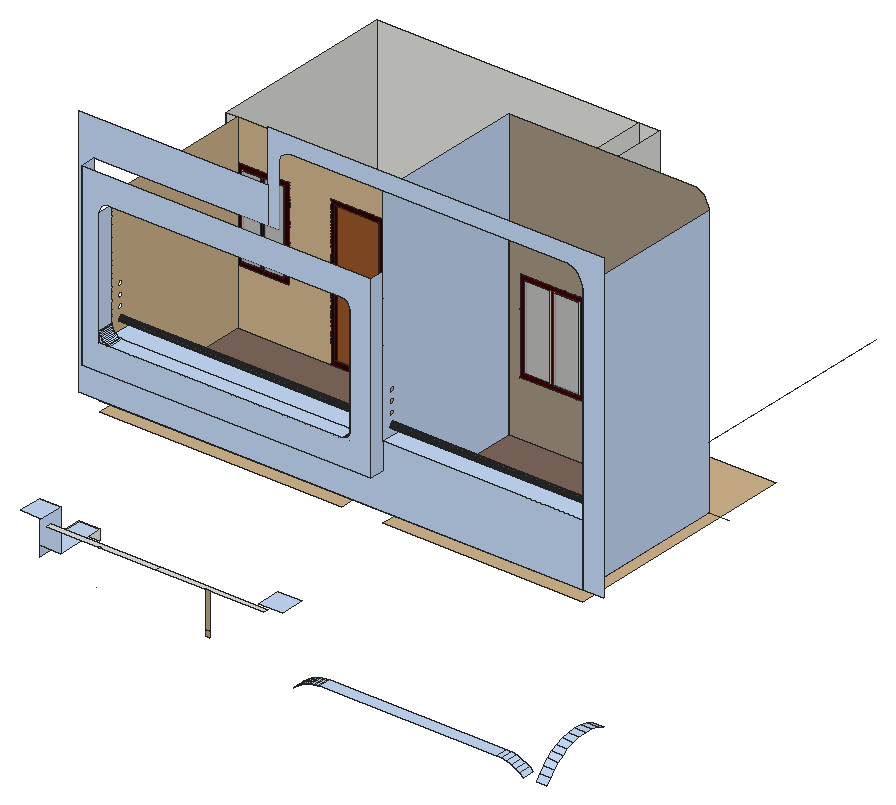
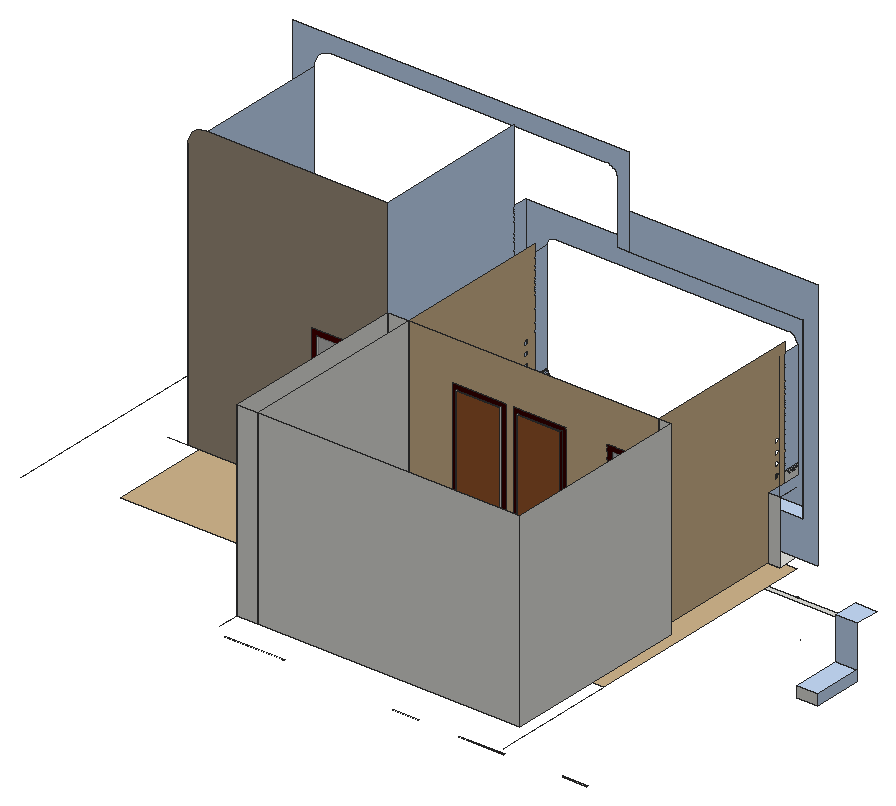
# SketchUp Ruby script. Lengths in inches.
U = 1.inch
M = Sketchup.active_model
def pt(a) = Geom::Point3d.new(a.map { |v| v * U })
def face(e, loops, mat)
  f = e.add_face(loops[0].map { |a| pt(a) })
  loops[1..].each { |l| e.add_face(l.map { |a| pt(a) }).erase! }
  f.material = f.back_material = mat if mat
  f
end
# faces: each face lists its corners as indices into pts; further lists are holes
def faces(e, pts, list, mat = nil) = list.each { |f| face(e, (f[0].is_a?(Array) ? f : [f]).map { |l| l.map { |i| pts[i] } }, mat) }
# xy, xz, yz: faces in a plane at the given z, y or x. An outline is a flat list of corners, or four numbers for a rectangle; further outlines are holes
def ring(l) = l.size == 4 ? [[l[0], l[1]], [l[2], l[1]], [l[2], l[3]], [l[0], l[3]]] : l.each_slice(2).to_a
def flat(e, list, mat, &to3) = list.each { |f| face(e, (f[0].is_a?(Array) ? f : [f]).map { |l| ring(l).map { |u, v| to3.(u, v) } }, mat) }
def xy(e, z, list, mat = nil) = flat(e, list, mat) { |x, y| [x, y, z] }
def xz(e, y, list, mat = nil) = flat(e, list, mat) { |x, z| [x, y, z] }
def yz(e, x, list, mat = nil) = flat(e, list, mat) { |y, z| [x, y, z] }
def lines(e, pts, list) = list.each { |a, b| e.add_line(pt(pts[a]), pt(pts[b])) }
# prism: a flat outline (further loops are holes) pulled along v
def prism(e, loops, v, mat = nil)
  f = face(e, loops, mat); d = Geom::Vector3d.new(v.map { |x| x * U })
  f.pushpull(f.normal.samedirection?(d) ? d.length : -d.length)
end
def box(e, o, s, mat = nil) = prism(e, [[o, [o[0] + s[0], o[1], o[2]], [o[0] + s[0], o[1] + s[1], o[2]], [o[0], o[1] + s[1], o[2]]]], [0, 0, s[2]], mat)
def at(x, y, z, deg = 0) = Geom::Transformation.translation(pt([x, y, z])) * Geom::Transformation.rotation(ORIGIN, Z_AXIS, deg.degrees)
def axes(o, x, y, z) = Geom::Transformation.new([*x, 0, *y, 0, *z, 0, *pt(o).to_a, 1])
def part(name) = M.definitions.add(name)
# library, detail: a bought-in or finely detailed component or shape, given as its bounding box
def library(name, o, s) = part(name).tap { |d| box(d.entities, o, s) }
def detail(e, o, s) = box(e.add_group.entities, o, s)
def put(e, d, t, mat = nil) = e.add_instance(d, t).tap { |i| i.material = mat if mat }
def group(e, t, mat = nil) = e.add_group.tap { |g| g.transformation = t; g.material = mat if mat }.entities
root = M.entities
M.materials.add("[0022_Maroon]").color = [56, 0, 0]
M.materials.add("[0022_Maroon]1").color = [71, 0, 0]
M.materials.add("[0033_NavajoWhite]").color = [209, 182, 141]
M.materials.add("[0033_NavajoWhite]1").color = [188, 164, 128]
M.materials.add("[0099_LightSteelBlue]").color = [198, 220, 249]
M.materials.add("[Cladding Siding Tan]").color = [162, 148, 128]
M.materials.add("[Granite Brown]").color = [126, 104, 91]
M.materials.add("[Metal Steel Textured White]").color = [84, 84, 84]
M.materials.add("[Translucent Resin Crush Gray]").color = [184, 184, 184]
M.materials["[Translucent Resin Crush Gray]"].alpha = 0.8
M.materials.add("[Wood Cherry Original]").color = [152, 86, 42]
xy(root,120,[[342.64,0,545.36,13.78]],"[0099_LightSteelBlue]")
xy(root,132,[[0,27.5625,24,84]],"[0099_LightSteelBlue]")
xy(root,143.8125,[[42.69,359,71.07,360],[236.63,359,265,360]])
xy(root,143.8125,[[137.32,360,188.45,361]],"[0022_Maroon]")
xy(root,152.24,[[388.21,360,456,361]])
xy(root,168,[[24,7.78,148.22,13.78],[148.22,7.78,272.4375,13.78]])
xy(root,180,[[0,0,24,27.5625],[272.4375,0,300,27.5625]],"[0099_LightSteelBlue]")
xy(root,252,[[82.32,129.1,79.97,129.1875,77.73,129.88,75.74,131.13,74.14,132.86,73.05,134.9375,72.53,137.23,72.62,139.58,73.31,141.82,74.57,143.81,76.29,145.4,78.37,146.5,80.66,147.02,83.01,146.93,85.25,146.23,87.24,144.98,88.84,143.26,89.93,141.18,90.45,138.89,90.36,136.54,89.67,134.3,88.41,132.31,86.69,130.71,84.61,129.62],[166.32,129.1,163.97,129.1875,161.73,129.88,159.74,131.13,158.14,132.86,157.05,134.9375,156.53,137.23,156.62,139.58,157.31,141.82,158.57,143.81,160.29,145.4,162.37,146.5,164.66,147.02,167.01,146.93,169.25,146.23,171.24,144.98,172.84,143.26,173.93,141.18,174.45,138.89,174.36,136.54,173.67,134.3,172.41,132.31,170.69,130.71,168.61,129.62],[250.32,129.1,247.97,129.1875,245.73,129.88,243.74,131.13,242.14,132.86,241.05,134.9375,240.53,137.23,240.62,139.58,241.31,141.82,242.57,143.81,244.29,145.4,246.37,146.5,248.66,147.02,251.01,146.93,253.25,146.23,255.24,144.98,256.84,143.26,257.93,141.18,258.45,138.89,258.36,136.54,257.67,134.3,256.41,132.31,254.69,130.71,252.61,129.62],[432.35,130.11,430.02,130.42,427.85,131.32,425.99,132.76,424.56,134.62,423.66,136.79,423.36,139.125,423.67,141.45,424.57,143.62,426,145.49,427.87,146.91,430.04,147.81,432.37,148.11,434.7,147.8,436.87,146.9,438.73,145.47,440.16,143.6,441.05,141.43,441.36,139.1,441.05,136.77,440.15,134.6,438.71,132.74,436.85,131.3125,434.68,130.42],[300,180,348,360]])
xy(root,252,[[[24,84,24,360,300,360,300,180,348,180,348,360,576,360,576,84,348,84,348,104.375,300,104.375,300,84],[166.32,129.1,168.61,129.62,170.69,130.71,172.41,132.31,173.67,134.3,174.36,136.54,174.45,138.89,173.93,141.18,172.84,143.26,171.24,144.98,169.25,146.23,167.01,146.93,164.66,147.02,162.37,146.5,160.29,145.4,158.57,143.81,157.31,141.82,156.62,139.58,156.53,137.23,157.05,134.9375,158.14,132.86,159.74,131.13,161.73,129.88,163.97,129.1875],[82.32,129.1,84.61,129.62,86.69,130.71,88.41,132.31,89.67,134.3,90.36,136.54,90.45,138.89,89.93,141.18,88.84,143.26,87.24,144.98,85.25,146.23,83.01,146.93,80.66,147.02,78.37,146.5,76.29,145.4,74.57,143.81,73.31,141.82,72.62,139.58,72.53,137.23,73.05,134.9375,74.14,132.86,75.74,131.13,77.73,129.88,79.97,129.1875],[250.32,129.1,252.61,129.62,254.69,130.71,256.41,132.31,257.67,134.3,258.36,136.54,258.45,138.89,257.93,141.18,256.84,143.26,255.24,144.98,253.25,146.23,251.01,146.93,248.66,147.02,246.37,146.5,244.29,145.4,242.57,143.81,241.31,141.82,240.62,139.58,240.53,137.23,241.05,134.9375,242.14,132.86,243.74,131.13,245.73,129.88,247.97,129.1875],[432.35,130.11,434.68,130.42,436.85,131.3125,438.71,132.74,440.15,134.6,441.05,136.77,441.36,139.1,441.05,141.43,440.16,143.6,438.73,145.47,436.87,146.9,434.7,147.8,432.37,148.11,430.04,147.81,427.87,146.91,426,145.49,424.57,143.62,423.67,141.45,423.36,139.125,423.66,136.79,424.56,134.62,425.99,132.76,427.85,131.32,430.02,130.42]]],"[0033_NavajoWhite]")
xy(root,264,[[24,84,576,108],[324,108,348,264],[24,264,324,480],[324,264,348,480]])
xy(root,264,[[37.43,108,324,264],[348,108,576,264]],"[Granite Brown]")
xy(root,269,[[148.81,264,198.81,266],[218.18,264,268.18,266]])
xy(root,306,[[17.11,66,348,84]],"[0099_LightSteelBlue]")
xy(root,332.63,[[366.6875,263,395.75,264],[399.75,263,428.8125,264]])
xy(root,334.32,[[43.43,263,65.05,264],[69.05,263,90.68,264]])
xy(root,336,[[37.43,66,49.21,84]])
xy(root,336,[[49.21,66,314.66,84],[37.43,84,324,108],[348,84,576,108]],"[0099_LightSteelBlue]")
xz(root,7.78,[[82.51,168,86.11,168,82.51,168.02]])
xz(root,7.78,[[210.33,120.05,210.33,126.08,209.08,126.22,205.44,126.24,205.44,120.25,208.74,120.23],[210.33,126.08,210.33,168,205.44,168,205.44,126.24,209.08,126.22]],"[0033_NavajoWhite]1")
xz(root,27.5625,[[0,132,24,180]],"[0099_LightSteelBlue]")
xz(root,66,[[[17.11,306,348,510],[37.43,336,37.43,469.26,37.52,470.66,37.79,472.04,38.24,473.37,38.86,474.63,39.64,475.8,40.57,476.85,41.625,477.78,42.79,478.5625,44.05,479.18,45.38,479.63,46.76,479.91,48.16,480,314.66,480,315.88,479.92,317.08,479.68,318.24,479.29,319.33,478.75,320.35,478.07,321.27,477.27,322.07,476.35,322.75,475.33,323.29,474.24,323.68,473.08,323.92,471.88,324,470.66,324,345.34,323.92,344.12,323.68,342.92,323.29,341.76,322.75,340.67,322.07,339.65,321.27,338.73,320.35,337.93,319.33,337.25,318.24,336.71,317.08,336.32,315.88,336.08,314.66,336]],[37.43,336,49.21,336,47.67,336.1,46.16,336.4,44.7,336.9,43.32,337.58,42.04,338.4375,40.88,339.45,39.86,340.61,39,341.89,38.32,343.28,37.83,344.74,37.53,346.25,37.43,347.79]],"[0099_LightSteelBlue]")
xz(root,84,[[0,120,24,132]])
xz(root,84,[[0,264,576,264,576,336,348,336,348,306,17.11,306,17.11,510,216,510,216,552,0,552],[576,264,600,264,600,612,216,612,216,510,228,510,228,577.99,228.13,579.93,228.51,581.84,229.13,583.68,229.99,585.42,231.07,587.04,232.35,588.5,233.8125,589.78,235.43,590.86,237.17,591.72,239.01,592.35,240.92,592.72,242.86,592.85,556.05,592.85,558.65,592.68,561.21,592.17,563.68,591.33,566.02,590.18,568.19,588.73,570.16,587.01,571.875,585.05,573.33,582.875,574.48,580.53,575.32,578.0625,575.83,575.5,576,572.9]],"[0099_LightSteelBlue]")
xz(root,108,[[24,264,37.43,336],[324,264,348,336],[348,264,576,336]])
xz(root,108,[[37.43,264,324,336]],"[0099_LightSteelBlue]")
xz(root,263,[[366.6875,332.63,395.75,427.88],[399.75,332.63,428.8125,427.88],[43.43,334.32,65.05,427.88],[69.05,334.32,90.68,427.88]],"[Translucent Resin Crush Gray]")
xz(root,264,[[24,264,37.43,480],[324,264,348,480]])
xz(root,264,[[[143.81,264,203.81,433.88],[148.81,269,198.81,428.88]],[[213.18,264,273.18,433.88],[218.18,269,268.18,428.88]],[[37.43,328.32,96.68,433.88],[43.43,334.32,90.68,427.88]],[65.05,334.32,69.05,427.88]],"[0022_Maroon]")
xz(root,264,[[[360.6875,326.63,434.8125,433.88],[366.6875,332.63,428.8125,427.88]],[395.75,332.63,399.75,427.88]],"[0022_Maroon]1")
xz(root,264,[[37.43,264,143.81,264,143.81,433.88,203.81,433.88,203.81,264,213.18,264,213.18,433.88,273.18,433.88,273.18,264,324,264,324,480,37.43,480,37.43,433.88,96.68,433.88,96.68,328.32,37.43,328.32]],"[0033_NavajoWhite]")
xz(root,264,[[[348,264,576,264,576,572.9,575.83,575.5,575.32,578.0625,574.48,580.53,573.33,582.875,571.875,585.05,570.16,587.01,568.19,588.73,566.02,590.18,563.68,591.33,561.21,592.17,558.65,592.68,556.05,592.85,348,592.85],[360.6875,326.63,434.8125,433.88]]],"[Cladding Siding Tan]")
xz(root,266,[[148.81,269,198.81,428.88],[218.18,269,268.18,428.88]],"[Wood Cherry Original]")
xz(root,480,[[24,264,324,480],[324,264,348,480]])
yz(root,0,[[27.5625,120,84,132]],"[0099_LightSteelBlue]")
yz(root,17.11,[[66,306,84,510]],"[0099_LightSteelBlue]")
yz(root,24,[[264,264,480,480]])
yz(root,37.43,[[66,336,84,347.79]])
yz(root,37.43,[[[108,264,264,264,264,480,84,480,84,336,108,336],[96,381,95.22,381.1,94.5,381.4,93.88,381.88,93.4,382.5,93.1,383.22,93,384,93.1,384.78,93.4,385.5,93.88,386.12,94.5,386.6,95.22,386.9,96,387,96.78,386.9,97.5,386.6,98.12,386.12,98.6,385.5,98.9,384.78,99,384,98.9,383.22,98.6,382.5,98.12,381.88,97.5,381.4,96.78,381.1],[96,369,95.22,369.1,94.5,369.4,93.88,369.88,93.4,370.5,93.1,371.22,93,372,93.1,372.78,93.4,373.5,93.88,374.12,94.5,374.6,95.22,374.9,96,375,96.78,374.9,97.5,374.6,98.12,374.12,98.6,373.5,98.9,372.78,99,372,98.9,371.22,98.6,370.5,98.12,369.88,97.5,369.4,96.78,369.1],[96,357,95.22,357.1,94.5,357.4,93.88,357.88,93.4,358.5,93.1,359.22,93,360,93.1,360.78,93.4,361.5,93.88,362.12,94.5,362.6,95.22,362.9,96,363,96.78,362.9,97.5,362.6,98.12,362.12,98.6,361.5,98.9,360.78,99,360,98.9,359.22,98.6,358.5,98.12,357.88,97.5,357.4,96.78,357.1],[96,345,95.22,345.1,94.5,345.4,93.88,345.88,93.4,346.5,93.1,347.22,93,348,93.1,348.78,93.4,349.5,93.88,350.12,94.5,350.6,95.22,350.9,96,351,96.78,350.9,97.5,350.6,98.12,350.12,98.6,349.5,98.9,348.78,99,348,98.9,347.22,98.6,346.5,98.12,345.88,97.5,345.4,96.78,345.1]]],"[0033_NavajoWhite]")
yz(root,37.43,[[66,347.79,84,469.26]],"[0099_LightSteelBlue]")
yz(root,43.43,[[263,334.32,264,427.88]])
yz(root,65.05,[[263,334.32,264,427.88]],"[0022_Maroon]")
yz(root,69.05,[[263,334.32,264,427.88]])
yz(root,90.68,[[263,334.32,264,427.88]],"[0022_Maroon]")
yz(root,148.81,[[264,269,266,428.88]],"[0022_Maroon]")
yz(root,198.81,[[264,269,266,428.88]])
yz(root,218.18,[[264,269,266,428.88]])
yz(root,268.18,[[264,269,266,428.88]])
yz(root,324,[[264,264,480,480],[96,345,96.78,345.1,97.5,345.4,98.12,345.88,98.6,346.5,98.9,347.22,99,348,98.9,348.78,98.6,349.5,98.12,350.12,97.5,350.6,96.78,350.9,96,351,95.22,350.9,94.5,350.6,93.88,350.12,93.4,349.5,93.1,348.78,93,348,93.1,347.22,93.4,346.5,93.88,345.88,94.5,345.4,95.22,345.1]])
yz(root,324,[[[108,264,108,336,84,336,84,480,264,480,264,264],[96,369,96.78,369.1,97.5,369.4,98.12,369.88,98.6,370.5,98.9,371.22,99,372,98.9,372.78,98.6,373.5,98.12,374.12,97.5,374.6,96.78,374.9,96,375,95.22,374.9,94.5,374.6,93.88,374.12,93.4,373.5,93.1,372.78,93,372,93.1,371.22,93.4,370.5,93.88,369.88,94.5,369.4,95.22,369.1],[96,357,96.78,357.1,97.5,357.4,98.12,357.88,98.6,358.5,98.9,359.22,99,360,98.9,360.78,98.6,361.5,98.12,362.12,97.5,362.6,96.78,362.9,96,363,95.22,362.9,94.5,362.6,93.88,362.12,93.4,361.5,93.1,360.78,93,360,93.1,359.22,93.4,358.5,93.88,357.88,94.5,357.4,95.22,357.1],[96,345,96.78,345.1,97.5,345.4,98.12,345.88,98.6,346.5,98.9,347.22,99,348,98.9,348.78,98.6,349.5,98.12,350.12,97.5,350.6,96.78,350.9,96,351,95.22,350.9,94.5,350.6,93.88,350.12,93.4,349.5,93.1,348.78,93,348,93.1,347.22,93.4,346.5,93.88,345.88,94.5,345.4,95.22,345.1],[96,381,96.78,381.1,97.5,381.4,98.12,381.88,98.6,382.5,98.9,383.22,99,384,98.9,384.78,98.6,385.5,98.12,386.12,97.5,386.6,96.78,386.9,96,387,95.22,386.9,94.5,386.6,93.88,386.12,93.4,385.5,93.1,384.78,93,384,93.1,383.22,93.4,382.5,93.88,381.88,94.5,381.4,95.22,381.1]]],"[0033_NavajoWhite]")
yz(root,324,[[66,345.34,84,470.66]],"[0099_LightSteelBlue]")
yz(root,348,[[264,264,480,480]])
yz(root,348,[[[108,264,264,264,264,592.85,84,592.85,84,336,108,336],[96,345,95.22,345.1,94.5,345.4,93.88,345.88,93.4,346.5,93.1,347.22,93,348,93.1,348.78,93.4,349.5,93.88,350.12,94.5,350.6,95.22,350.9,96,351,96.78,350.9,97.5,350.6,98.12,350.12,98.6,349.5,98.9,348.78,99,348,98.9,347.22,98.6,346.5,98.12,345.88,97.5,345.4,96.78,345.1],[96,369,95.22,369.1,94.5,369.4,93.88,369.88,93.4,370.5,93.1,371.22,93,372,93.1,372.78,93.4,373.5,93.88,374.12,94.5,374.6,95.22,374.9,96,375,96.78,374.9,97.5,374.6,98.12,374.12,98.6,373.5,98.9,372.78,99,372,98.9,371.22,98.6,370.5,98.12,369.88,97.5,369.4,96.78,369.1],[96,357,95.22,357.1,94.5,357.4,93.88,357.88,93.4,358.5,93.1,359.22,93,360,93.1,360.78,93.4,361.5,93.88,362.12,94.5,362.6,95.22,362.9,96,363,96.78,362.9,97.5,362.6,98.12,362.12,98.6,361.5,98.9,360.78,99,360,98.9,359.22,98.6,358.5,98.12,357.88,97.5,357.4,96.78,357.1],[96,381,95.22,381.1,94.5,381.4,93.88,381.88,93.4,382.5,93.1,383.22,93,384,93.1,384.78,93.4,385.5,93.88,386.12,94.5,386.6,95.22,386.9,96,387,96.78,386.9,97.5,386.6,98.12,386.12,98.6,385.5,98.9,384.78,99,384,98.9,383.22,98.6,382.5,98.12,381.88,97.5,381.4,96.78,381.1]],[66,306,84,510]],"[0099_LightSteelBlue]")
yz(root,366.6875,[[263,332.63,264,427.88]])
yz(root,395.75,[[263,332.63,264,427.88]])
yz(root,399.75,[[263,332.63,264,427.88]])
yz(root,428.8125,[[263,332.63,264,427.88]])
yz(root,576,[[84,264,108,336],[96,345,96.78,345.1,97.5,345.4,98.12,345.88,98.6,346.5,98.9,347.22,99,348,98.9,348.78,98.6,349.5,98.12,350.12,97.5,350.6,96.78,350.9,96,351,95.22,350.9,94.5,350.6,93.88,350.12,93.4,349.5,93.1,348.78,93,348,93.1,347.22,93.4,346.5,93.88,345.88,94.5,345.4,95.22,345.1]])
yz(root,576,[[[108,264,108,336,84,336,84,572.9,264,572.9,264,264],[96,381,96.78,381.1,97.5,381.4,98.12,381.88,98.6,382.5,98.9,383.22,99,384,98.9,384.78,98.6,385.5,98.12,386.12,97.5,386.6,96.78,386.9,96,387,95.22,386.9,94.5,386.6,93.88,386.12,93.4,385.5,93.1,384.78,93,384,93.1,383.22,93.4,382.5,93.88,381.88,94.5,381.4,95.22,381.1],[96,369,96.78,369.1,97.5,369.4,98.12,369.88,98.6,370.5,98.9,371.22,99,372,98.9,372.78,98.6,373.5,98.12,374.12,97.5,374.6,96.78,374.9,96,375,95.22,374.9,94.5,374.6,93.88,374.12,93.4,373.5,93.1,372.78,93,372,93.1,371.22,93.4,370.5,93.88,369.88,94.5,369.4,95.22,369.1],[96,357,96.78,357.1,97.5,357.4,98.12,357.88,98.6,358.5,98.9,359.22,99,360,98.9,360.78,98.6,361.5,98.12,362.12,97.5,362.6,96.78,362.9,96,363,95.22,362.9,94.5,362.6,93.88,362.12,93.4,361.5,93.1,360.78,93,360,93.1,359.22,93.4,358.5,93.88,357.88,94.5,357.4,95.22,357.1],[96,345,96.78,345.1,97.5,345.4,98.12,345.88,98.6,346.5,98.9,347.22,99,348,98.9,348.78,98.6,349.5,98.12,350.12,97.5,350.6,96.78,350.9,96,351,95.22,350.9,94.5,350.6,93.88,350.12,93.4,349.5,93.1,348.78,93,348,93.1,347.22,93.4,346.5,93.88,345.88,94.5,345.4,95.22,345.1]]],"[0099_LightSteelBlue]")
p = [[600,3.51,106.92],[600,7.87,113.24],[588,7.87,113.24],[588,3.51,106.92],[314.11,13.78,109.05],[312.49,13.78,107.51],
  [312.49,0,107.51],[314.11,0,109.05],[575.51,13.78,107.51],[571.32,13.78,111.1875],[571.32,0,111.1875],[575.51,0,107.51],
  [315.81,13.78,110.5],[315.81,0,110.5],[317.58,13.78,111.86],[317.58,0,111.86],[566.68,13.78,114.29],[566.68,0,114.29],
  [319.42,13.78,113.12],[319.42,0,113.12],[321.32,13.78,114.29],[321.32,0,114.29],[600,12.96,118.98],[588,12.96,118.98],
  [323.28,13.78,115.35],[323.28,0,115.35],[561.68,13.78,116.75],[561.68,0,116.75],[325.3,13.78,116.3125],[325.3,0,116.3125],
  [327.36,13.78,117.17],[327.36,0,117.17],[556.4,13.78,118.55],[556.4,0,118.55],[329.46,13.78,117.91],[329.46,0,117.91],
  [331.6,13.78,118.55],[331.6,0,118.55],[333.78,13.78,119.07],[333.78,0,119.07],[550.92,13.78,119.64],[550.92,0,119.64],
  [600,18.7,124.07],[588,18.7,124.07],[588,13.78,119.71],[335.97,13.78,119.48],[335.97,0,119.48],[338.18,13.78,119.77],
  [338.18,0,119.77],[545.36,13.78,120],[545.36,0,120],[340.41,13.78,119.94],[340.41,0,119.94],[342.64,13.78,120],
  [342.64,0,120],[600,25.02,128.43],[588,25.02,128.43],[600,31.8125,132],[588,31.8125,132],[600,40.22,135.09],
  [588,40.22,135.09],[600,75.6,135.09],[600,84,132],[588,84,132],[588,75.6,135.09],[600,48.97,136.97],
  [588,48.97,136.97],[600,66.84,136.97],[588,66.84,136.97],[600,57.91,137.6],[588,57.91,137.6],[49.21,84,336],
  [47.67,84,336.1],[47.67,66,336.1],[49.21,66,336],[315.88,84,336.08],[314.66,84,336],[314.66,66,336],
  [315.88,66,336.08],[46.16,84,336.4],[46.16,66,336.4],[317.08,84,336.32],[317.08,66,336.32],[318.24,84,336.71],
  [318.24,66,336.71],[44.7,84,336.9],[44.7,66,336.9],[319.33,84,337.25],[319.33,66,337.25],[43.32,84,337.58],
  [43.32,66,337.58],[320.35,84,337.93],[320.35,66,337.93],[42.04,84,338.4375],[42.04,66,338.4375],[321.27,84,338.73],
  [321.27,66,338.73],[40.88,84,339.45],[40.88,66,339.45],[322.07,84,339.65],[322.07,66,339.65],[39.86,84,340.61],
  [39.86,66,340.61],[322.75,84,340.67],[322.75,66,340.67],[39,84,341.89],[39,66,341.89],[323.29,84,341.76],
  [323.29,66,341.76],[323.68,84,342.92],[323.68,66,342.92],[38.32,84,343.28],[38.32,66,343.28],[323.92,84,344.12],
  [323.92,66,344.12],[37.83,84,344.74],[37.83,66,344.74],[324,84,345.34],[324,66,345.34],[37.53,84,346.25],
  [37.53,66,346.25],[324,96,345],[324,95.22,345.1],[37.43,95.22,345.1],[37.43,96,345],[576,96,345],
  [576,95.22,345.1],[348,95.22,345.1],[348,96,345],[324,96.78,345.1],[37.43,96.78,345.1],[576,96.78,345.1],
  [348,96.78,345.1],[324,94.5,345.4],[37.43,94.5,345.4],[576,94.5,345.4],[348,94.5,345.4],[324,97.5,345.4],
  [37.43,97.5,345.4],[576,97.5,345.4],[348,97.5,345.4],[324,93.88,345.88],[37.43,93.88,345.88],[576,93.88,345.88],
  [348,93.88,345.88],[324,98.12,345.88],[37.43,98.12,345.88],[576,98.12,345.88],[348,98.12,345.88],[324,93.4,346.5],
  [37.43,93.4,346.5],[576,93.4,346.5],[348,93.4,346.5],[324,98.6,346.5],[37.43,98.6,346.5],[576,98.6,346.5],
  [348,98.6,346.5],[37.43,84,347.79],[37.43,66,347.79],[324,93.1,347.22],[37.43,93.1,347.22],[576,93.1,347.22],
  [348,93.1,347.22],[324,98.9,347.22],[37.43,98.9,347.22],[576,98.9,347.22],[348,98.9,347.22],[324,93,348],
  [37.43,93,348],[576,93,348],[348,93,348],[324,99,348],[37.43,99,348],[576,99,348],
  [348,99,348],[324,93.1,348.78],[37.43,93.1,348.78],[576,93.1,348.78],[348,93.1,348.78],[324,98.9,348.78],
  [37.43,98.9,348.78],[576,98.9,348.78],[348,98.9,348.78],[324,93.4,349.5],[37.43,93.4,349.5],[576,93.4,349.5],
  [348,93.4,349.5],[324,98.6,349.5],[37.43,98.6,349.5],[576,98.6,349.5],[348,98.6,349.5],[324,93.88,350.12],
  [37.43,93.88,350.12],[576,93.88,350.12],[348,93.88,350.12],[324,98.12,350.12],[37.43,98.12,350.12],[576,98.12,350.12],
  [348,98.12,350.12],[324,94.5,350.6],[37.43,94.5,350.6],[576,94.5,350.6],[348,94.5,350.6],[324,97.5,350.6],
  [37.43,97.5,350.6],[576,97.5,350.6],[348,97.5,350.6],[324,95.22,350.9],[37.43,95.22,350.9],[576,95.22,350.9],
  [348,95.22,350.9],[324,96.78,350.9],[37.43,96.78,350.9],[576,96.78,350.9],[348,96.78,350.9],[324,96,351],
  [37.43,96,351],[576,96,351],[348,96,351],[24,360,252],[24,504,252],[576,264,264],
  [600,264,264],[24,108,336],[24,108,480],[24,84,336],[324,84,336],[324,66,336],
  [348,504,264],[348,480,264],[576,264,336],[576,504,336],[37.43,96,348],[324,96,348],
  [348,96,348],[576,96,348],[80.89,7.78,125.88],[80.89,7.78,126.18]]
faces(root,p,[[0,1,2,3],[4,5,6,7],[8,9,10,11],[12,4,7,13],[14,12,13,15],[9,16,17,10],[18,14,15,19],[20,18,19,21],
  [1,22,23,2],[24,20,21,25],[16,26,27,17],[28,24,25,29],[30,28,29,31],[26,32,33,27],[34,30,31,35],[36,34,35,37],
  [38,36,37,39],[32,40,41,33],[22,42,43,44,23],[45,38,39,46],[47,45,46,48],[40,49,50,41],[51,47,48,52],[53,51,52,54],
  [42,55,56,43],[55,57,58,56],[57,59,60,58],[61,62,63,64],[59,65,66,60],[67,61,64,68],[65,69,70,66],[69,67,68,70],
  [71,72,73,74],[75,76,77,78],[72,79,80,73],[81,75,78,82],[83,81,82,84],[79,85,86,80],[87,83,84,88],[85,89,90,86],
  [91,87,88,92],[89,93,94,90],[95,91,92,96],[93,97,98,94],[99,95,96,100],[97,101,102,98],[103,99,100,104],[101,105,106,102],
  [107,103,104,108],[109,107,108,110],[105,111,112,106],[113,109,110,114],[111,115,116,112],[117,113,114,118],[115,119,120,116],[119,157,158,120]],"[0099_LightSteelBlue]")
faces(root,p,[[121,122,123,124],[125,126,127,128],[129,121,124,130],[131,125,128,132],[122,133,134,123],[126,135,136,127],[137,129,130,138],[139,131,132,140],
  [133,141,142,134],[135,143,144,136],[145,137,138,146],[147,139,140,148],[141,149,150,142],[143,151,152,144],[153,145,146,154],[155,147,148,156],
  [149,159,160,150],[151,161,162,152],[163,153,154,164],[165,155,156,166],[159,167,168,160],[161,169,170,162],[171,163,164,172],[173,165,166,174],
  [167,175,176,168],[169,177,178,170],[179,171,172,180],[181,173,174,182],[175,183,184,176],[177,185,186,178],[187,179,180,188],[189,181,182,190],
  [183,191,192,184],[185,193,194,186],[195,187,188,196],[197,189,190,198],[191,199,200,192],[193,201,202,194],[203,195,196,204],[205,197,198,206],
  [199,207,208,200],[201,209,210,202],[211,203,204,212],[213,205,206,214],[207,215,216,208],[209,217,218,210],[215,211,212,216],[217,213,214,218]],"[Metal Steel Textured White]")
lines(root,p,[[219,220],[221,222],[223,224],[223,225],[226,227],[228,229],[230,231],[232,124],[233,232],[234,128],[235,234],[218,234],
  [216,232],[236,237]])
